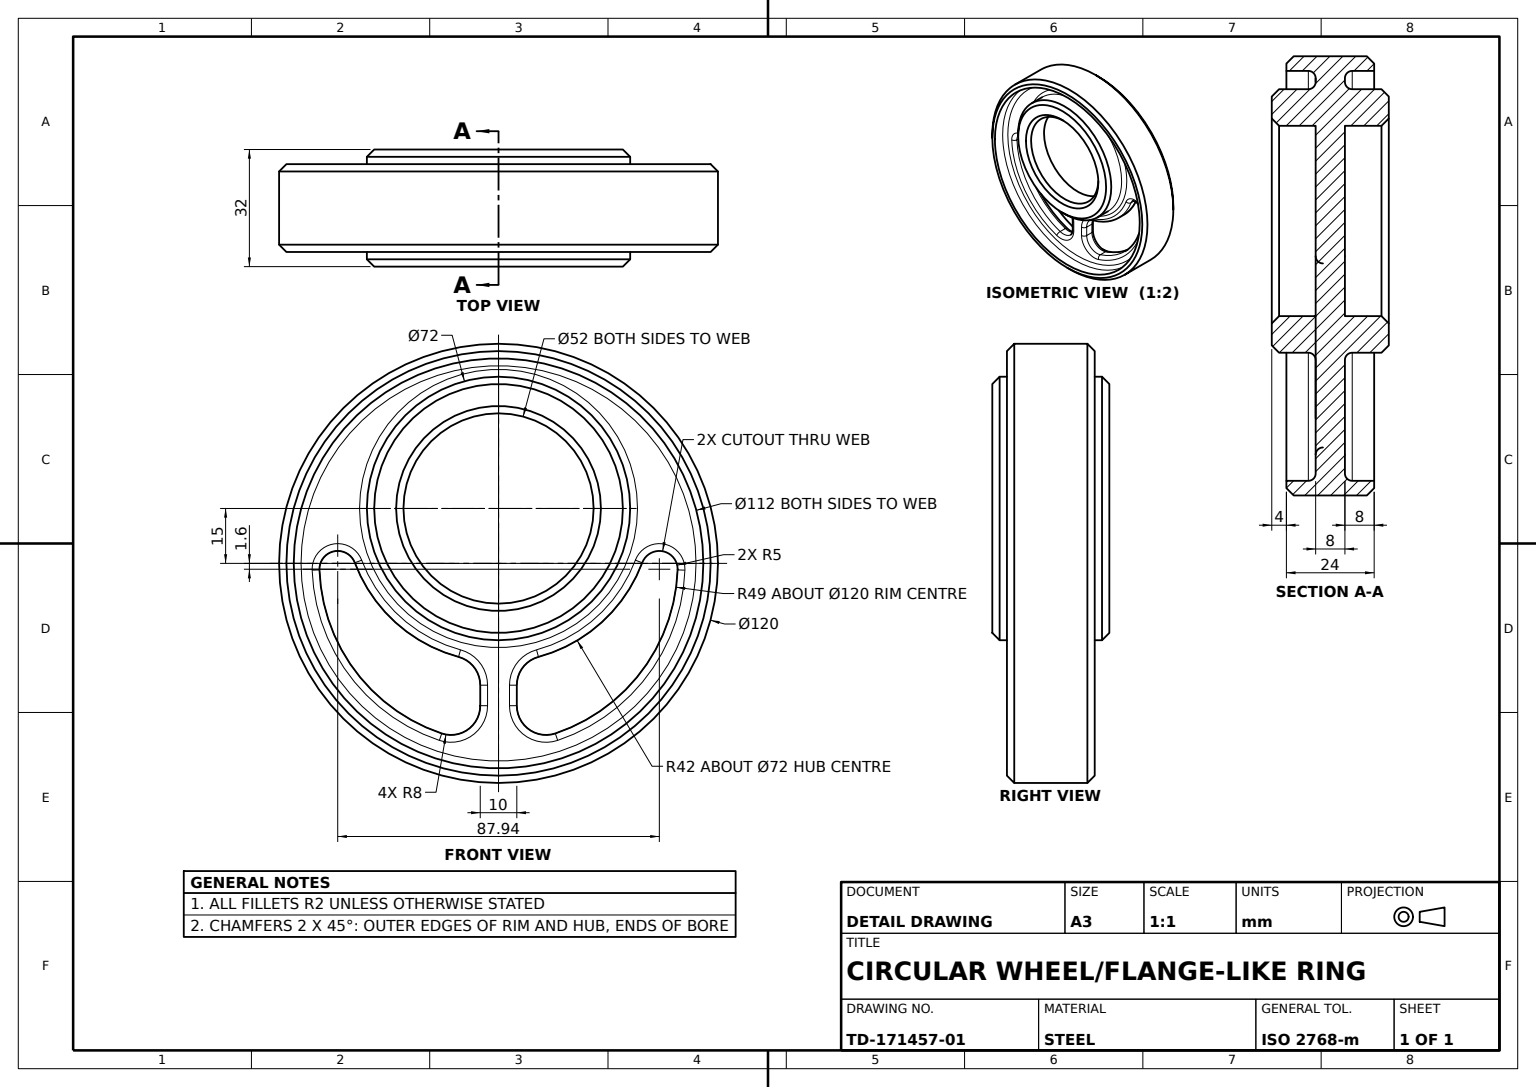
solid
v1 (-10.4,23.624345,4)
v2 (-37.422042,-0.87234,4)
e1 v1 v2 CIRCLE(AX(P(0,-15,4),D(0,0,1),D(1,0,0)),40)
v3 (-10.92,25.555562,2)
e2 v1 v3 CIRCLE(AX(P(-10.4,23.624345,2),D(-0.965608616,-0.26,0),D(0.26,-0.965608616,0)),2)
v4 (-39.293144,-0.165957,2)
e3 v4 v3 CIRCLE(AX(P(0,-15,2),D(0,0,-1),D(1,0,0)),42)
e4 v2 v4 CIRCLE(AX(P(-37.422042,-0.87234,2),D(-0.353191489,-0.935551053,0),D(0.935551053,-0.353191489,0)),2)
face TORUS(AX(P(0,-15,2),D(0,0,1),D(1,0,0)),40,2) [-e1 e2 -e3 -e4]
v5 (56,0,6)
v6 (-56,0,6)
e5 v5 v6 CIRCLE(AX(P(0,0,6),D(0,0,-1),D(1,0,0)),56)
v7 (-56,0,12)
e6 v7 v6 LINE
v8 (56,0,12)
e7 v7 v8 CIRCLE(AX(P(0,0,12),D(0,0,1),D(1,0,0)),56)
e8 v8 v5 LINE
face CYL(AX(P(0,0,12),D(0,0,-1),D(-1,0,0)),56) rev [e5 -e6 e7 e8]
v9 (-5,38.884444,2)
v10 (-15.536585,46.471653,2)
e9 v9 v10 CIRCLE(AX(P(-13,38.884444,2),D(0,0,1),D(1,0,0)),8)
v11 (-15.536585,46.471653,-2)
e10 v11 v10 LINE
v12 (-5,38.884444,-2)
e11 v11 v12 CIRCLE(AX(P(-13,38.884444,-2),D(0,0,-1),D(1,0,0)),8)
e12 v12 v9 LINE
face CYL(AX(P(-13,38.884444,-17),D(0,0,1),D(1,0,0)),8) rev [e9 -e10 e11 e12]
v13 (-16.170732,48.368455,4)
v14 (-3,38.884444,4)
e13 v13 v14 CIRCLE(AX(P(-13,38.884444,4),D(0,0,-1),D(1,0,0)),10)
e14 v10 v13 CIRCLE(AX(P(-16.170732,48.368455,2),D(-0.948401078,-0.317073171,0),D(0.317073171,-0.948401078,0)),2)
e15 v9 v14 CIRCLE(AX(P(-3,38.884444,2),D(0,1,0),D(0,0,1)),2)
face TORUS(AX(P(-13,38.884444,2),D(0,0,1),D(1,0,0)),10,2) [-e13 -e14 -e9 e15]
v15 (36,-15,-6)
v16 (36,-15,-14)
e16 v15 v16 LINE
v17 (-36,-15,-14)
e17 v16 v17 CIRCLE(AX(P(0,-15,-14),D(0,0,1),D(1,0,0)),36)
v18 (-36,-15,-6)
e18 v18 v17 LINE
e19 v18 v15 CIRCLE(AX(P(0,-15,-6),D(0,0,-1),D(1,0,0)),36)
face CYL(AX(P(0,-15,16),D(0,0,-1),D(-1,0,0)),36) [e16 e17 -e18 e19]
v19 (36,-15,14)
v20 (-36,-15,14)
e20 v19 v20 CIRCLE(AX(P(0,-15,14),D(0,0,-1),D(1,0,0)),36)
v21 (34,-15,16)
e21 v21 v19 LINE
v22 (-34,-15,16)
e22 v22 v21 CIRCLE(AX(P(0,-15,16),D(0,0,1),D(1,0,0)),34)
e23 v22 v20 LINE
face CONE(AX(P(0,-15,16),D(0,0,-1),D(-1,0,0)),34,0.785398163) [-e20 -e21 -e22 e23]
v23 (26,-15,4)
v24 (-26,-15,4)
e24 v23 v24 CIRCLE(AX(P(0,-15,4),D(0,0,-1),D(1,0,0)),26)
e25 v24 v23 CIRCLE(AX(P(0,-15,4),D(0,0,-1),D(1,0,0)),26)
face PLANE(AX(P(0,0,4),D(0,0,1),D(1,0,0))) [-e24 -e25]
v25 (-5,33.280431,2)
e26 v3 v25 CIRCLE(AX(P(-13,33.280431,2),D(0,0,1),D(1,0,0)),8)
v26 (-5,33.280431,-2)
e27 v26 v25 LINE
v27 (-10.92,25.555562,-2)
e28 v26 v27 CIRCLE(AX(P(-13,33.280431,-2),D(0,0,-1),D(1,0,0)),8)
e29 v27 v3 LINE
face CYL(AX(P(-13,33.280431,-17),D(0,0,1),D(1,0,0)),8) rev [e26 -e27 e28 e29]
v28 (3,38.884444,-4)
v29 (3,33.280431,-4)
e30 v28 v29 LINE
v30 (5,38.884444,-2)
e31 v30 v28 CIRCLE(AX(P(3,38.884444,-2),D(0,1,0),D(0,0,1)),2)
v31 (5,33.280431,-2)
e32 v31 v30 LINE
e33 v29 v31 CIRCLE(AX(P(3,33.280431,-2),D(0,-1,0),D(0,0,-1)),2)
face CYL(AX(P(3,0,-2),D(0,-1,0),D(0,0,-1)),2) [-e30 -e31 -e32 -e33]
e34 v17 v16 CIRCLE(AX(P(0,-15,-14),D(0,0,1),D(1,0,0)),36)
v32 (-34,-15,-16)
e35 v32 v17 LINE
v33 (34,-15,-16)
e36 v33 v32 CIRCLE(AX(P(0,-15,-16),D(0,0,-1),D(1,0,0)),34)
e37 v33 v16 LINE
face CONE(AX(P(0,-15,-14),D(0,0,1),D(1,0,0)),36,0.785398163) [-e34 -e35 -e36 e37]
v34 (-48.967593,1.781818,2)
e38 v10 v34 CIRCLE(AX(P(0,0,2),D(0,0,1),D(1,0,0)),49)
v35 (-50.96627,1.854545,4)
e39 v35 v13 CIRCLE(AX(P(0,0,4),D(0,0,-1),D(1,0,0)),51)
e40 v35 v34 CIRCLE(AX(P(-50.96627,1.854545,2),D(0.036363636,0.999338624,0),D(-0.999338624,0.036363636,0)),2)
face TORUS(AX(P(0,0,2),D(0,0,1),D(1,0,0)),51,2) [-e38 e14 -e39 e40]
v36 (-56,0,-6)
v37 (56,0,-6)
e41 v36 v37 CIRCLE(AX(P(0,0,-6),D(0,0,1),D(1,0,0)),56)
v38 (56,0,-12)
e42 v37 v38 LINE
v39 (-56,0,-12)
e43 v39 v38 CIRCLE(AX(P(0,0,-12),D(0,0,1),D(1,0,0)),56)
e44 v36 v39 LINE
face CYL(AX(P(0,0,12),D(0,0,-1),D(-1,0,0)),56) rev [e41 e42 -e43 -e44]
v40 (48.967593,1.781818,-2)
v41 (48.970899,1.6,-2)
e45 v40 v41 CIRCLE(AX(P(43.970899,1.6,-2),D(0,0,-1),D(1,0,0)),5)
v42 (50.96627,1.854545,-4)
e46 v40 v42 CIRCLE(AX(P(50.96627,1.854545,-2),D(0.036363636,-0.999338624,0),D(0.999338624,0.036363636,0)),2)
v43 (50.970899,1.6,-4)
e47 v43 v42 CIRCLE(AX(P(43.970899,1.6,-4),D(0,0,1),D(1,0,0)),7)
e48 v41 v43 CIRCLE(AX(P(50.970899,1.6,-2),D(0,-1,0),D(0,0,-1)),2)
face TORUS(AX(P(43.970899,1.6,-2),D(0,0,1),D(1,0,0)),7,2) [-e45 e46 -e47 -e48]
v44 (-60,0,-10)
v45 (60,0,-10)
e49 v44 v45 CIRCLE(AX(P(0,0,-10),D(0,0,1),D(1,0,0)),60)
v46 (60,0,10)
e50 v46 v45 LINE
v47 (-60,0,10)
e51 v46 v47 CIRCLE(AX(P(0,0,10),D(0,0,-1),D(1,0,0)),60)
e52 v47 v44 LINE
face CYL(AX(P(0,0,12),D(0,0,-1),D(-1,0,0)),60) [e49 -e50 e51 e52]
v48 (-54,0,-4)
e53 v36 v48 CIRCLE(AX(P(-54,0,-6),D(0,1,0),D(-1,0,0)),2)
e54 v37 v36 CIRCLE(AX(P(0,0,-6),D(0,0,1),D(1,0,0)),56)
v49 (54,0,-4)
e55 v37 v49 CIRCLE(AX(P(54,0,-6),D(0,-1,0),D(0,0,-1)),2)
e56 v48 v49 CIRCLE(AX(P(0,0,-4),D(0,0,-1),D(1,0,0)),54)
face TORUS(AX(P(0,0,-6),D(0,0,1),D(1,0,0)),54,2) rev [-e53 -e54 e55 -e56]
v50 (-26,-15,14)
v51 (26,-15,14)
e57 v50 v51 CIRCLE(AX(P(0,-15,14),D(0,0,1),D(1,0,0)),26)
v52 (-28,-15,16)
e58 v50 v52 LINE
v53 (28,-15,16)
e59 v53 v52 CIRCLE(AX(P(0,-15,16),D(0,0,-1),D(1,0,0)),28)
e60 v51 v53 LINE
face CONE(AX(P(0,-15,14),D(0,0,1),D(1,0,0)),26,0.785398163) rev [-e57 e58 -e59 -e60]
v54 (48.967593,1.781818,2)
v55 (50.96627,1.854545,4)
e61 v54 v55 CIRCLE(AX(P(50.96627,1.854545,2),D(-0.036363636,0.999338624,0),D(-0.999338624,-0.036363636,0)),2)
v56 (16.170732,48.368455,4)
e62 v56 v55 CIRCLE(AX(P(0,0,4),D(0,0,-1),D(1,0,0)),51)
v57 (15.536585,46.471653,2)
e63 v57 v56 CIRCLE(AX(P(16.170732,48.368455,2),D(-0.948401078,0.317073171,0),D(-0.317073171,-0.948401078,0)),2)
e64 v54 v57 CIRCLE(AX(P(0,0,2),D(0,0,1),D(1,0,0)),49)
face TORUS(AX(P(0,0,2),D(0,0,1),D(1,0,0)),51,2) [e61 -e62 -e63 -e64]
v58 (58,0,12)
e65 v58 v46 LINE
v59 (-58,0,12)
e66 v59 v58 CIRCLE(AX(P(0,0,12),D(0,0,1),D(1,0,0)),58)
e67 v59 v47 LINE
face CONE(AX(P(0,0,12),D(0,0,-1),D(-1,0,0)),58,0.785398163) [-e65 -e66 e67 -e51]
e68 v51 v50 CIRCLE(AX(P(0,-15,14),D(0,0,1),D(1,0,0)),26)
e69 v52 v53 CIRCLE(AX(P(0,-15,16),D(0,0,-1),D(1,0,0)),28)
face CONE(AX(P(0,-15,14),D(0,0,1),D(1,0,0)),26,0.785398163) rev [-e58 -e68 e60 -e69]
v60 (15.536585,46.471653,-2)
e70 v60 v40 CIRCLE(AX(P(0,0,-2),D(0,0,-1),D(1,0,0)),49)
e71 v40 v54 LINE
e72 v60 v57 LINE
face CYL(AX(P(0,0,-17),D(0,0,1),D(1,0,0)),49) rev [e70 e71 e64 -e72]
v61 (-3,33.280431,4)
e73 v14 v61 LINE
e74 v25 v9 LINE
e75 v25 v61 CIRCLE(AX(P(-3,33.280431,2),D(0,1,0),D(0,0,1)),2)
face CYL(AX(P(-3,0,2),D(0,-1,0),D(0,0,-1)),2) [-e73 -e15 -e74 e75]
v62 (-39.293144,-0.165957,-2)
e76 v62 v4 LINE
e77 v27 v62 CIRCLE(AX(P(0,-15,-2),D(0,0,1),D(1,0,0)),42)
face CYL(AX(P(0,-15,-17),D(0,0,1),D(1,0,0)),42) [e76 e3 -e29 e77]
e78 v12 v26 LINE
face PLANE(AX(P(-5,0,-17),D(-1,0,0),D(0,0,1))) [-e12 e78 e27 e74]
v63 (16.170732,48.368455,-4)
e79 v63 v28 CIRCLE(AX(P(13,38.884444,-4),D(0,0,1),D(1,0,0)),10)
e80 v60 v63 CIRCLE(AX(P(16.170732,48.368455,-2),D(0.948401078,-0.317073171,0),D(0.317073171,0.948401078,0)),2)
e81 v30 v60 CIRCLE(AX(P(13,38.884444,-2),D(0,0,-1),D(1,0,0)),8)
face TORUS(AX(P(13,38.884444,-2),D(0,0,1),D(1,0,0)),10,2) [-e79 -e80 -e81 e31]
v64 (-36,-15,6)
e82 v20 v64 LINE
e83 v20 v19 CIRCLE(AX(P(0,-15,14),D(0,0,-1),D(1,0,0)),36)
v65 (36,-15,6)
e84 v19 v65 LINE
e85 v65 v64 CIRCLE(AX(P(0,-15,6),D(0,0,1),D(1,0,0)),36)
face CYL(AX(P(0,-15,16),D(0,0,-1),D(-1,0,0)),36) [-e82 e83 e84 e85]
e86 v51 v23 LINE
e87 v50 v24 LINE
face CYL(AX(P(0,-15,16),D(0,0,-1),D(-1,0,0)),26) rev [e86 e24 -e87 e57]
v66 (5,38.884444,2)
e88 v57 v66 CIRCLE(AX(P(13,38.884444,2),D(0,0,1),D(1,0,0)),8)
e89 v30 v66 LINE
face CYL(AX(P(13,38.884444,-17),D(0,0,1),D(1,0,0)),8) rev [e88 -e89 e81 e72]
e90 v64 v65 CIRCLE(AX(P(0,-15,6),D(0,0,1),D(1,0,0)),36)
face CYL(AX(P(0,-15,16),D(0,0,-1),D(-1,0,0)),36) [-e84 e20 e82 e90]
e91 v61 v1 CIRCLE(AX(P(-13,33.280431,4),D(0,0,-1),D(1,0,0)),10)
face TORUS(AX(P(-13,33.280431,2),D(0,0,1),D(1,0,0)),10,2) [-e91 -e75 -e26 -e2]
v67 (-16.170732,48.368455,-4)
e92 v11 v67 CIRCLE(AX(P(-16.170732,48.368455,-2),D(0.948401078,0.317073171,0),D(-0.317073171,0.948401078,0)),2)
v68 (-3,38.884444,-4)
e93 v68 v67 CIRCLE(AX(P(-13,38.884444,-4),D(0,0,1),D(1,0,0)),10)
e94 v12 v68 CIRCLE(AX(P(-3,38.884444,-2),D(0,-1,0),D(0,0,-1)),2)
face TORUS(AX(P(-13,38.884444,-2),D(0,0,1),D(1,0,0)),10,2) [e92 -e93 -e94 -e11]
v69 (-37.422042,-0.87234,-4)
e95 v69 v62 CIRCLE(AX(P(-37.422042,-0.87234,-2),D(0.353191489,0.935551053,0),D(-0.935551053,0.353191489,0)),2)
v70 (-10.4,23.624345,-4)
e96 v70 v27 CIRCLE(AX(P(-10.4,23.624345,-2),D(0.965608616,0.26,0),D(-0.26,0.965608616,0)),2)
e97 v69 v70 CIRCLE(AX(P(0,-15,-4),D(0,0,-1),D(1,0,0)),40)
face TORUS(AX(P(0,-15,-2),D(0,0,1),D(1,0,0)),40,2) [e95 -e77 -e96 -e97]
v71 (39.293144,-0.165957,-2)
v72 (39.293144,-0.165957,2)
e98 v71 v72 LINE
v73 (48.970899,1.6,2)
e99 v72 v73 CIRCLE(AX(P(43.970899,1.6,2),D(0,0,1),D(1,0,0)),5)
e100 v41 v73 LINE
e101 v41 v71 CIRCLE(AX(P(43.970899,1.6,-2),D(0,0,-1),D(1,0,0)),5)
face CYL(AX(P(43.970899,1.6,-17),D(0,0,1),D(1,0,0)),5) rev [e98 e99 -e100 e101]
v74 (-58,0,-12)
e102 v74 v44 LINE
v75 (58,0,-12)
e103 v75 v74 CIRCLE(AX(P(0,0,-12),D(0,0,-1),D(1,0,0)),58)
e104 v75 v45 LINE
face CONE(AX(P(0,0,-10),D(0,0,1),D(1,0,0)),60,0.785398163) [-e49 -e102 -e103 e104]
e105 v49 v48 CIRCLE(AX(P(0,0,-4),D(0,0,-1),D(1,0,0)),54)
v76 (10.4,23.624345,-4)
e106 v29 v76 CIRCLE(AX(P(13,33.280431,-4),D(0,0,1),D(1,0,0)),10)
v77 (37.422042,-0.87234,-4)
e107 v76 v77 CIRCLE(AX(P(0,-15,-4),D(0,0,-1),D(1,0,0)),40)
e108 v77 v43 CIRCLE(AX(P(43.970899,1.6,-4),D(0,0,1),D(1,0,0)),7)
e109 v42 v63 CIRCLE(AX(P(0,0,-4),D(0,0,1),D(1,0,0)),51)
v78 (38,-15,-4)
v79 (-38,-15,-4)
e110 v78 v79 CIRCLE(AX(P(0,-15,-4),D(0,0,1),D(1,0,0)),38)
e111 v79 v78 CIRCLE(AX(P(0,-15,-4),D(0,0,1),D(1,0,0)),38)
v80 (-50.96627,1.854545,-4)
e112 v67 v80 CIRCLE(AX(P(0,0,-4),D(0,0,1),D(1,0,0)),51)
e113 v80 v69 CIRCLE(AX(P(-43.970899,1.6,-4),D(0,0,1),D(1,0,0)),7)
v81 (-3,33.280431,-4)
e114 v70 v81 CIRCLE(AX(P(-13,33.280431,-4),D(0,0,1),D(1,0,0)),10)
e115 v81 v68 LINE
face PLANE(AX(P(0,0,-4),D(0,0,1),D(1,0,0))) rev [e105 e56] [e79 e30 e106 e107 e108 e47 e109] [e110 e111] [e112 e113 e97 e114 e115 e93]
e116 v15 v18 CIRCLE(AX(P(0,-15,-6),D(0,0,-1),D(1,0,0)),36)
face CYL(AX(P(0,-15,16),D(0,0,-1),D(-1,0,0)),36) [e18 e34 -e16 e116]
e117 v8 v7 CIRCLE(AX(P(0,0,12),D(0,0,1),D(1,0,0)),56)
e118 v6 v5 CIRCLE(AX(P(0,0,6),D(0,0,-1),D(1,0,0)),56)
face CYL(AX(P(0,0,12),D(0,0,-1),D(-1,0,0)),56) rev [-e8 e117 e6 e118]
e119 v32 v33 CIRCLE(AX(P(0,-15,-16),D(0,0,-1),D(1,0,0)),34)
v82 (-28,-15,-16)
v83 (28,-15,-16)
e120 v82 v83 CIRCLE(AX(P(0,-15,-16),D(0,0,1),D(1,0,0)),28)
e121 v83 v82 CIRCLE(AX(P(0,-15,-16),D(0,0,1),D(1,0,0)),28)
face PLANE(AX(P(0,0,-16),D(0,0,1),D(1,0,0))) rev [e36 e119] [e120 e121]
v84 (-26,-15,-4)
v85 (26,-15,-4)
e122 v84 v85 CIRCLE(AX(P(0,-15,-4),D(0,0,-1),D(1,0,0)),26)
v86 (-26,-15,-14)
e123 v84 v86 LINE
v87 (26,-15,-14)
e124 v86 v87 CIRCLE(AX(P(0,-15,-14),D(0,0,-1),D(1,0,0)),26)
e125 v85 v87 LINE
face CYL(AX(P(0,-15,16),D(0,0,-1),D(-1,0,0)),26) rev [-e122 e123 e124 -e125]
v88 (5,33.280431,2)
e126 v31 v88 LINE
e127 v66 v88 LINE
face PLANE(AX(P(5,0,-17),D(-1,0,0),D(0,0,1))) rev [-e126 e32 e89 e127]
e128 v21 v22 CIRCLE(AX(P(0,-15,16),D(0,0,1),D(1,0,0)),34)
face PLANE(AX(P(0,0,16),D(0,0,1),D(1,0,0))) [e22 e128] [e69 e59]
e129 v34 v4 CIRCLE(AX(P(-43.970899,1.6,2),D(0,0,1),D(1,0,0)),5)
v89 (-48.967593,1.781818,-2)
e130 v62 v89 CIRCLE(AX(P(-43.970899,1.6,-2),D(0,0,-1),D(1,0,0)),5)
e131 v89 v34 LINE
face CYL(AX(P(-43.970899,1.6,-17),D(0,0,1),D(1,0,0)),5) rev [e129 -e76 e130 e131]
v90 (-38,-15,4)
v91 (38,-15,4)
e132 v90 v91 CIRCLE(AX(P(0,-15,4),D(0,0,-1),D(1,0,0)),38)
e133 v64 v90 CIRCLE(AX(P(-38,-15,6),D(0,1,0),D(-1,0,0)),2)
e134 v65 v91 CIRCLE(AX(P(38,-15,6),D(0,-1,0),D(0,0,-1)),2)
face TORUS(AX(P(0,-15,6),D(0,0,1),D(1,0,0)),38,2) rev [-e132 -e133 -e85 e134]
e135 v91 v90 CIRCLE(AX(P(0,-15,4),D(0,0,-1),D(1,0,0)),38)
face TORUS(AX(P(0,-15,6),D(0,0,1),D(1,0,0)),38,2) rev [-e135 -e134 -e90 e133]
e136 v78 v15 CIRCLE(AX(P(38,-15,-6),D(0,-1,0),D(0,0,-1)),2)
e137 v79 v18 CIRCLE(AX(P(-38,-15,-6),D(0,1,0),D(-1,0,0)),2)
face TORUS(AX(P(0,-15,-6),D(0,0,1),D(1,0,0)),38,2) rev [e136 -e19 -e137 -e110]
e138 v45 v44 CIRCLE(AX(P(0,0,-10),D(0,0,1),D(1,0,0)),60)
e139 v47 v46 CIRCLE(AX(P(0,0,10),D(0,0,-1),D(1,0,0)),60)
face CYL(AX(P(0,0,12),D(0,0,-1),D(-1,0,0)),60) [e138 -e52 e139 e50]
e140 v2 v35 CIRCLE(AX(P(-43.970899,1.6,4),D(0,0,-1),D(1,0,0)),7)
face TORUS(AX(P(-43.970899,1.6,2),D(0,0,1),D(1,0,0)),7,2) [e4 -e129 -e40 -e140]
v92 (10.92,25.555562,-2)
v93 (10.92,25.555562,2)
e141 v92 v93 LINE
e142 v92 v31 CIRCLE(AX(P(13,33.280431,-2),D(0,0,-1),D(1,0,0)),8)
e143 v88 v93 CIRCLE(AX(P(13,33.280431,2),D(0,0,1),D(1,0,0)),8)
face CYL(AX(P(13,33.280431,-17),D(0,0,1),D(1,0,0)),8) rev [-e141 e142 e126 e143]
e144 v26 v81 CIRCLE(AX(P(-3,33.280431,-2),D(0,-1,0),D(0,0,-1)),2)
face TORUS(AX(P(-13,33.280431,-2),D(0,0,1),D(1,0,0)),10,2) [-e114 e96 -e28 e144]
face CYL(AX(P(-3,0,-2),D(0,1,0),D(0,0,1)),2) [-e78 e94 -e115 -e144]
e145 v73 v54 CIRCLE(AX(P(43.970899,1.6,2),D(0,0,1),D(1,0,0)),5)
face CYL(AX(P(43.970899,1.6,-17),D(0,0,1),D(1,0,0)),5) rev [-e71 e45 e100 e145]
face CONE(AX(P(0,-15,16),D(0,0,-1),D(-1,0,0)),34,0.785398163) [-e128 e21 -e83 -e23]
e146 v38 v39 CIRCLE(AX(P(0,0,-12),D(0,0,1),D(1,0,0)),56)
face CYL(AX(P(0,0,12),D(0,0,-1),D(-1,0,0)),56) rev [e44 -e146 -e42 e54]
e147 v85 v84 CIRCLE(AX(P(0,-15,-4),D(0,0,-1),D(1,0,0)),26)
e148 v87 v86 CIRCLE(AX(P(0,-15,-14),D(0,0,-1),D(1,0,0)),26)
face CYL(AX(P(0,-15,16),D(0,0,-1),D(-1,0,0)),26) rev [-e123 -e147 e125 e148]
e149 v87 v83 LINE
e150 v86 v82 LINE
face CONE(AX(P(0,-15,-16),D(0,0,-1),D(-1,0,0)),28,0.785398163) rev [e149 -e120 -e150 -e148]
e151 v89 v11 CIRCLE(AX(P(0,0,-2),D(0,0,-1),D(1,0,0)),49)
face CYL(AX(P(0,0,-17),D(0,0,1),D(1,0,0)),49) rev [e151 e10 e38 -e131]
v94 (10.4,23.624345,4)
e152 v94 v93 CIRCLE(AX(P(10.4,23.624345,2),D(-0.965608616,0.26,0),D(-0.26,-0.965608616,0)),2)
v95 (3,33.280431,4)
e153 v95 v88 CIRCLE(AX(P(3,33.280431,2),D(0,1,0),D(0,0,1)),2)
e154 v94 v95 CIRCLE(AX(P(13,33.280431,4),D(0,0,-1),D(1,0,0)),10)
face TORUS(AX(P(13,33.280431,2),D(0,0,1),D(1,0,0)),10,2) [e152 -e143 -e153 -e154]
v96 (54,0,4)
e155 v96 v5 CIRCLE(AX(P(54,0,6),D(0,-1,0),D(0,0,-1)),2)
v97 (-54,0,4)
e156 v97 v96 CIRCLE(AX(P(0,0,4),D(0,0,1),D(1,0,0)),54)
e157 v97 v6 CIRCLE(AX(P(-54,0,6),D(0,1,0),D(-1,0,0)),2)
face TORUS(AX(P(0,0,6),D(0,0,1),D(1,0,0)),54,2) rev [-e5 -e155 -e156 e157]
e158 v93 v72 CIRCLE(AX(P(0,-15,2),D(0,0,-1),D(1,0,0)),42)
v98 (37.422042,-0.87234,4)
e159 v98 v94 CIRCLE(AX(P(0,-15,4),D(0,0,1),D(1,0,0)),40)
e160 v98 v72 CIRCLE(AX(P(37.422042,-0.87234,2),D(-0.353191489,0.935551053,0),D(-0.935551053,-0.353191489,0)),2)
face TORUS(AX(P(0,-15,2),D(0,0,1),D(1,0,0)),40,2) [-e158 -e152 -e159 e160]
face PLANE(AX(P(0,0,-4),D(0,0,1),D(1,0,0))) rev [e122 e147]
e161 v80 v89 CIRCLE(AX(P(-50.96627,1.854545,-2),D(-0.036363636,-0.999338624,0),D(0.999338624,-0.036363636,0)),2)
face TORUS(AX(P(0,0,-2),D(0,0,1),D(1,0,0)),51,2) [-e112 -e92 -e151 -e161]
v99 (50.970899,1.6,4)
e162 v99 v98 CIRCLE(AX(P(43.970899,1.6,4),D(0,0,-1),D(1,0,0)),7)
e163 v99 v73 CIRCLE(AX(P(50.970899,1.6,2),D(0,-1,0),D(0,0,-1)),2)
face TORUS(AX(P(43.970899,1.6,2),D(0,0,1),D(1,0,0)),7,2) [-e99 -e160 -e162 e163]
face CONE(AX(P(0,-15,-16),D(0,0,-1),D(-1,0,0)),28,0.785398163) rev [e150 -e121 -e149 -e124]
face TORUS(AX(P(0,-15,-6),D(0,0,1),D(1,0,0)),38,2) rev [-e116 -e136 -e111 e137]
v100 (3,38.884444,4)
e164 v66 v100 CIRCLE(AX(P(3,38.884444,2),D(0,-1,0),D(0,0,-1)),2)
e165 v95 v100 LINE
face CYL(AX(P(3,0,2),D(0,1,0),D(0,0,1)),2) [e164 -e165 e153 -e127]
e166 v76 v92 CIRCLE(AX(P(10.4,23.624345,-2),D(0.965608616,-0.26,0),D(0.26,0.965608616,0)),2)
face TORUS(AX(P(13,33.280431,-2),D(0,0,1),D(1,0,0)),10,2) [-e166 -e106 e33 -e142]
e167 v55 v99 CIRCLE(AX(P(43.970899,1.6,4),D(0,0,-1),D(1,0,0)),7)
face TORUS(AX(P(43.970899,1.6,2),D(0,0,1),D(1,0,0)),7,2) [-e163 -e167 -e61 -e145]
e168 v58 v59 CIRCLE(AX(P(0,0,12),D(0,0,1),D(1,0,0)),58)
face CONE(AX(P(0,0,12),D(0,0,-1),D(-1,0,0)),58,0.785398163) [-e67 -e168 e65 -e139]
e169 v100 v56 CIRCLE(AX(P(13,38.884444,4),D(0,0,-1),D(1,0,0)),10)
e170 v96 v97 CIRCLE(AX(P(0,0,4),D(0,0,1),D(1,0,0)),54)
face PLANE(AX(P(0,0,4),D(0,0,1),D(1,0,0))) [e132 e135] [e165 e169 e62 e167 e162 e159 e154] [e140 e39 e13 e73 e91 e1] [e170 e156]
e171 v77 v71 CIRCLE(AX(P(37.422042,-0.87234,-2),D(0.353191489,-0.935551053,0),D(0.935551053,0.353191489,0)),2)
face TORUS(AX(P(43.970899,1.6,-2),D(0,0,1),D(1,0,0)),7,2) [e171 -e101 e48 -e108]
face CYL(AX(P(0,-15,16),D(0,0,-1),D(-1,0,0)),26) rev [e68 e87 e25 -e86]
face CONE(AX(P(0,-15,-14),D(0,0,1),D(1,0,0)),36,0.785398163) [-e37 -e119 e35 -e17]
e172 v74 v75 CIRCLE(AX(P(0,0,-12),D(0,0,-1),D(1,0,0)),58)
face CONE(AX(P(0,0,-10),D(0,0,1),D(1,0,0)),60,0.785398163) [-e172 e102 -e138 -e104]
e173 v71 v92 CIRCLE(AX(P(0,-15,-2),D(0,0,1),D(1,0,0)),42)
face CYL(AX(P(0,-15,-17),D(0,0,1),D(1,0,0)),42) [e173 e141 e158 -e98]
face TORUS(AX(P(0,0,-6),D(0,0,1),D(1,0,0)),54,2) rev [-e55 -e41 e53 -e105]
face TORUS(AX(P(-43.970899,1.6,-2),D(0,0,1),D(1,0,0)),7,2) [e161 -e130 -e95 -e113]
face TORUS(AX(P(0,-15,-2),D(0,0,1),D(1,0,0)),40,2) [-e171 -e107 e166 -e173]
face PLANE(AX(P(0,0,12),D(0,0,1),D(1,0,0))) [e168 e66] [-e117 -e7]
face TORUS(AX(P(0,0,-2),D(0,0,1),D(1,0,0)),51,2) [-e46 -e70 e80 -e109]
face TORUS(AX(P(13,38.884444,2),D(0,0,1),D(1,0,0)),10,2) [-e164 -e88 e63 -e169]
face TORUS(AX(P(0,0,6),D(0,0,1),D(1,0,0)),54,2) rev [e155 -e118 -e157 -e170]
face PLANE(AX(P(0,0,-12),D(0,0,1),D(1,0,0))) rev [e172 e103] [e43 e146]
